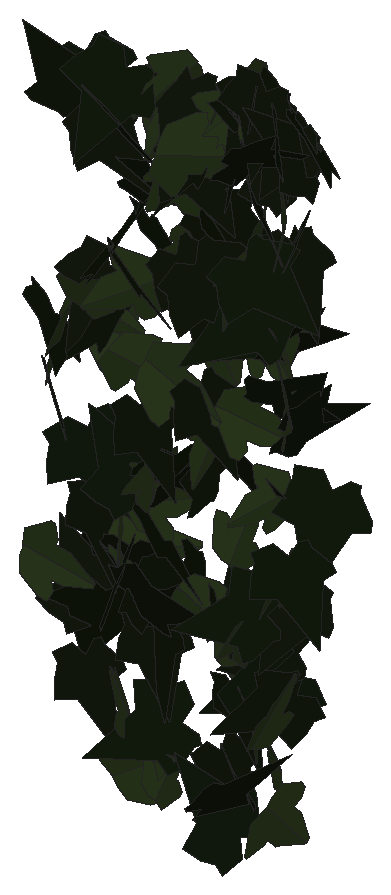
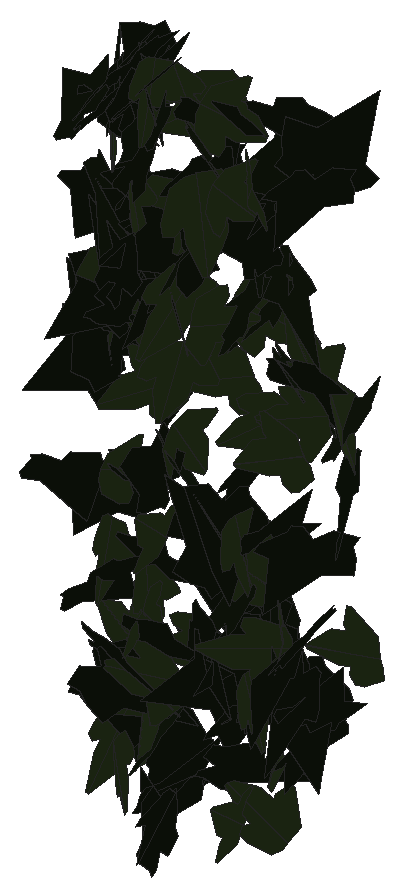
# SketchUp Ruby script. Lengths in inches.
U = 1.inch
M = Sketchup.active_model
def pt(a) = Geom::Point3d.new(a.map { |v| v * U })
def face(e, loops, mat)
  f = e.add_face(loops[0].map { |a| pt(a) })
  loops[1..].each { |l| e.add_face(l.map { |a| pt(a) }).erase! }
  f.material = f.back_material = mat if mat
  f
end
# faces: each face lists its corners as indices into pts; further lists are holes
def faces(e, pts, list, mat = nil) = list.each { |f| face(e, (f[0].is_a?(Array) ? f : [f]).map { |l| l.map { |i| pts[i] } }, mat) }
# xy, xz, yz: faces in a plane at the given z, y or x. An outline is a flat list of corners, or four numbers for a rectangle; further outlines are holes
def ring(l) = l.size == 4 ? [[l[0], l[1]], [l[2], l[1]], [l[2], l[3]], [l[0], l[3]]] : l.each_slice(2).to_a
def flat(e, list, mat, &to3) = list.each { |f| face(e, (f[0].is_a?(Array) ? f : [f]).map { |l| ring(l).map { |u, v| to3.(u, v) } }, mat) }
def xy(e, z, list, mat = nil) = flat(e, list, mat) { |x, y| [x, y, z] }
def xz(e, y, list, mat = nil) = flat(e, list, mat) { |x, z| [x, y, z] }
def yz(e, x, list, mat = nil) = flat(e, list, mat) { |y, z| [x, y, z] }
def lines(e, pts, list) = list.each { |a, b| e.add_line(pt(pts[a]), pt(pts[b])) }
# prism: a flat outline (further loops are holes) pulled along v
def prism(e, loops, v, mat = nil)
  f = face(e, loops, mat); d = Geom::Vector3d.new(v.map { |x| x * U })
  f.pushpull(f.normal.samedirection?(d) ? d.length : -d.length)
end
def box(e, o, s, mat = nil) = prism(e, [[o, [o[0] + s[0], o[1], o[2]], [o[0] + s[0], o[1] + s[1], o[2]], [o[0], o[1] + s[1], o[2]]]], [0, 0, s[2]], mat)
def at(x, y, z, deg = 0) = Geom::Transformation.translation(pt([x, y, z])) * Geom::Transformation.rotation(ORIGIN, Z_AXIS, deg.degrees)
def axes(o, x, y, z) = Geom::Transformation.new([*x, 0, *y, 0, *z, 0, *pt(o).to_a, 1])
def part(name) = M.definitions.add(name)
# library, detail: a bought-in or finely detailed component or shape, given as its bounding box
def library(name, o, s) = part(name).tap { |d| box(d.entities, o, s) }
def detail(e, o, s) = box(e.add_group.entities, o, s)
def put(e, d, t, mat = nil) = e.add_instance(d, t).tap { |i| i.material = mat if mat }
def group(e, t, mat = nil) = e.add_group.tap { |g| g.transformation = t; g.material = mat if mat }.entities
root = M.entities
M.materials.add("efeu1").color = [18, 25, 13]
M.materials.add("efeu2").color = [43, 57, 29]
c1 = part("ivyleaf_10")
p = [[0,0.5,-0.03],[-0.0625,2.02,-0.43],[-0.19,2.01,-0.46],[-0.54,1.05,-0.29],[-0.52,0.625,-0.18],[-0.83,0.76,-0.28],
  [-1.16,0.64,-0.33],[-1.15,0.33,-0.24],[-0.77,-0.39,0.02],[-0.3,-0.51,0.16],[0.04,-0.48,0.23],[-0.02,2.01,-0.4375],
  [-0.06,2.01,-0.43],[0.04,-0.49,0.23],[0.67,-0.49,0.14],[1.38,0.36,-0.2],[1.375,0.51,-0.24],[0.81,0.65,-0.19],
  [0.62,0.59,-0.15],[0.6,1.09,-0.28],[0.5,1.23,-0.31]]
faces(c1.entities,p,[[0,1,2,3,4,5,6,7,8,9,10],[11,12,0,13,14,15,16,17,18,19,20]],"efeu2")
c2 = part("ivyleaf_9")
p = [[1.54,2.16,1.25],[1.36,2.04,1.19],[-0.21,0.99,0.68],[-0.71,1.11,0.82],[-0.85,0.86,0.67],[-0.8,0.17,0.21],
  [-0.9,-0.01,0.1],[-0.67,-0.16,-0.02],[-0.08,-0.08,-0.05],[-0.03,-0.6,-0.4],[0.65,-0.88,-0.66],[0.83,-0.6,-0.49],
  [1.29,-0.42,-0.43],[1.8125,-0.07,-0.26],[1.21,0.44,0.15]]
faces(c2.entities,p,[[0,1,2,3,4,5,6,7,8,9,10,11,12,13,14]],"efeu1")
put(root,c1,axes([549.88,130.77,187.67],[0.2153,-0.80851,0.35731],[-0.00069,0.3676,0.83222],[-0.88394,-0.19722,0.08638]))
put(root,c1,axes([547.04,130.43,204.73],[-0.20339,-0.20216,-0.98043],[0.68566,0.7008,-0.28674],[0.72937,-0.71518,-0.00384]))
put(root,c2,axes([549.13,130.38,205.09],[0.50092,0.40394,0.56191],[0.37323,0.42644,-0.63928],[-0.58276,0.62033,0.07357]))
put(root,c2,axes([549.27,130.88,201.89],[0.22034,-0.57747,-0.68822],[0.24519,0.72037,-0.52594],[0.86429,-0.05715,0.32466]))
put(root,c1,axes([548.82,131.4375,201.4],[0.08871,-0.87143,0.33371],[0.0443,-0.3309,-0.87588],[0.93209,0.09866,0.00987]))
put(root,c2,axes([544.45,131.53,205.83],[-0.79635,-0.51494,-0.12466],[0.10914,0.06079,-0.9483],[0.51845,-0.80376,0.00814]))
put(root,c2,axes([545.1,131.28,190.01],[0.3464,-0.25474,0.81027],[0.68502,-0.43358,-0.42917],[0.50218,0.76717,0.02651]))
put(root,c1,axes([545.3,131.52,199.64],[-0.3442,-0.26523,0.88729],[-0.66707,-0.58559,-0.43382],[0.64237,-0.75023,0.02493]))
put(root,c2,axes([547.65,130.77,201.22],[0.25471,-0.54872,-0.85661],[-0.15872,0.8508,-0.59219],[1.00483,0.27348,0.12359]))
put(root,c1,axes([541.84,131.04,190.28],[0.12516,0.04099,0.9297],[0.89154,0.26368,-0.13165],[-0.26682,0.90027,-0.00377]))
put(root,c2,axes([549.41,131.61,200.25],[-0.90769,-0.27954,0.29998],[-0.2875,-0.08564,-0.94975],[0.29235,-0.95213,-0.00265]))
put(root,c2,axes([548.01,130.67,184.86],[0.23325,0.84885,-0.28298],[0.07285,0.27345,0.88031],[0.89181,-0.24435,0.0021]))
put(root,c2,axes([545,130.55,190.61],[-0.37818,0.2782,-0.85775],[-0.74103,0.4341,0.46752],[0.5138,0.83085,0.04294]))
put(root,c2,axes([549.31,131.46,190.83],[-0.72889,0.02884,0.51759],[-0.51813,-0.01249,-0.72896],[-0.01627,-0.89388,0.02688]))
put(root,c2,axes([548.41,131.43,183.8125],[-0.39425,-0.86849,0.10666],[0.04381,0.09724,0.95379],[-0.87392,0.39667,-0.00031]))
put(root,c1,axes([550.44,130.87,203.55],[0.30747,-0.52133,-0.65044],[-0.24336,0.60694,-0.6015],[0.79727,0.38631,0.06725]))
put(root,c2,axes([544.68,131.05,200.38],[0.77502,-0.30093,-0.2517],[-0.22074,0.12624,-0.83061],[0.32433,0.80503,0.03616]))
put(root,c2,axes([541.79,131.87,197.27],[0.09632,-0.66808,0.62784],[0.21106,-0.59818,-0.6689],[0.89217,0.21364,0.09046]))
put(root,c1,axes([542.41,131.48,197.52],[0.48601,-0.8469,0.10006],[0.04659,-0.08863,-0.97644],[0.85152,0.48823,-0.00368]))
put(root,c2,axes([542.375,130.99,195.75],[0.50052,-0.12141,-0.68792],[-0.66934,0.15881,-0.51503],[0.19989,0.83579,-0.00207]))
put(root,c1,axes([545.95,131.18,197.21],[0.38154,0.15398,0.97579],[0.92976,0.2975,-0.41049],[-0.33382,1.00461,-0.028]))
put(root,c1,axes([550.09,130.9,185.3],[-0.19039,-0.733,-0.64026],[0.21689,0.60404,-0.75602],[0.94878,-0.28517,0.04434]))
put(root,c2,axes([543.29,131.4,187.43],[0.1866,-0.78798,-0.33888],[-0.06518,0.33277,-0.80968],[0.85528,0.19728,0.01223]))
put(root,c2,axes([547.3,131.29,197.09],[0.28273,-0.72917,-0.45243],[-0.1741,0.4177,-0.78201],[0.84028,0.33189,-0.00979]))
put(root,c2,axes([546.625,131.21,200.97],[0.39542,-0.67732,-0.47211],[-0.03229,0.51038,-0.75926],[0.82499,0.34461,0.19657]))
put(root,c1,axes([549.73,131.8125,197.36],[-0.18437,0.10656,0.9668],[0.80848,-0.5303,0.21262],[0.54077,0.82915,0.01174]))
put(root,c2,axes([543.78,131.36,204.5625],[0.88461,-0.46342,0.30091],[0.27313,-0.12703,-0.99855],[0.48032,0.92572,0.01362]))
put(root,c2,axes([542.91,131.59,204.49],[0.49586,0.00518,0.83387],[-0.83093,0.08462,0.49359],[-0.07009,-0.96646,0.04768]))
put(root,c1,axes([544.48,131.53,186.14],[-0.56021,0.64858,0.27437],[0.17947,-0.20754,0.85703],[0.68098,0.58826,-0.00015]))
put(root,c1,axes([543.27,131.49,198.29],[-0.63726,-0.24393,0.44855],[0.46566,0.01659,0.67059],[-0.20943,0.77912,0.12616]))
put(root,c2,axes([544.67,131.16,200.98],[-0.53449,0.90076,-0.00372],[0.00008,-0.00428,-1.0474],[-0.90076,-0.53449,0.00211]))
put(root,c2,axes([550.14,131.55,192.79],[-0.3432,-0.4281,-0.67532],[0.45291,0.50155,-0.54811],[0.65893,-0.5677,0.02501]))
put(root,c1,axes([544.55,131.43,184.31],[-0.49014,-0.18346,0.74154],[0.69282,0.26435,0.52334],[-0.32176,0.84867,-0.00272]))
put(root,c2,axes([548.77,132.23,202.43],[-0.31713,-0.08599,1.04204],[0.23641,-1.06661,-0.01607],[1.0185,0.2208,0.32819]))
put(root,c2,axes([545.875,132.1,186.03],[-0.69274,-0.27828,0.53933],[-0.48329,-0.2421,-0.74568],[0.36708,-0.8439,0.03607]))
put(root,c2,axes([544,131.72,198.49],[-0.86008,0.45628,-0.14401],[0.12256,-0.07625,-0.97357],[-0.46251,-0.86871,0.00981]))
put(root,c1,axes([547.84,131.66,205.57],[0.64046,-0.17967,-0.51993],[-0.51041,0.10351,-0.6645],[0.20516,0.81841,-0.0301]))
put(root,c2,axes([546.96,131.82,204.26],[-0.75488,0.2554,-0.26246],[0.23738,-0.11666,-0.79624],[-0.27887,-0.79065,0.0327]))
put(root,c1,axes([548.64,131.59,190.27],[0.03476,-0.82313,-0.19316],[-0.01652,0.19263,-0.82382],[0.84532,0.03761,-0.00815]))
put(root,c2,axes([543.53,131.6,204.11],[0.32362,-0.67478,-0.53496],[-0.04206,0.55842,-0.72982],[0.86008,0.28121,0.16559]))
put(root,c2,axes([544.89,131.8,195.45],[0.28439,-0.79283,-0.3611],[-0.13006,0.33696,-0.84226],[0.86143,0.31262,-0.00795]))
put(root,c2,axes([549.26,132.36,204.55],[0.01543,-0.12146,0.89187],[0.09367,-0.88694,-0.12241],[0.89522,0.0949,-0.00256]))
put(root,c2,axes([548.2,132.23,205.79],[-0.50467,0.10336,-0.86624],[0.80917,-0.31856,-0.50943],[-0.32605,-0.95057,0.07653]))
put(root,c2,axes([544.53,131.875,192.98],[-0.48463,-0.68658,0.17349],[0.0965,0.14423,0.84038],[-0.70156,0.49412,-0.00424]))
put(root,c1,axes([547.04,132.26,195.52],[-0.08739,-0.70219,0.49403],[0.16901,-0.50094,-0.68211],[0.84177,0.02768,0.18824]))
put(root,c2,axes([548.6,132.42,206.16],[-0.08248,-0.86156,0.18638],[0.00251,-0.18743,-0.86527],[0.88149,-0.08008,0.0199]))
put(root,c2,axes([548.85,132.1,198.96],[0.44175,-0.55624,0.5064],[-0.31219,0.39873,0.71031],[-0.68438,-0.54093,0.00285]))
put(root,c2,axes([547.6875,131.42,199.9],[0.05818,-0.19803,-0.85883],[-0.2863,0.80977,-0.20612],[0.83357,0.29195,-0.01086]))
put(root,c2,axes([549.31,131.99,197.12],[0.88785,0.35219,-0.14803],[0.12722,0.08058,0.95475],[0.36023,-0.89649,0.02766]))
put(root,c1,axes([548.97,132.56,193.92],[-0.15855,-0.1143,0.80153],[-0.07362,-0.81134,-0.13026],[0.80629,-0.09655,0.14573]))
put(root,c2,axes([543.57,131.875,189.3125],[0.44343,0.65671,-0.6723],[-0.37509,-0.55794,-0.7924],[-0.86172,0.5808,-0.00104]))
put(root,c1,axes([543.57,132.52,190.8],[-0.13446,0.2921,-0.82646],[0.3256,-0.75965,-0.32146],[-0.81384,-0.35218,0.00793]))
put(root,c1,axes([545.66,132.58,205.78],[-0.09236,-0.50742,0.7116],[-0.17013,-0.69144,-0.51512],[0.85727,-0.19189,-0.02556]))
put(root,c1,axes([549.45,131.98,199.77],[-0.61986,-0.61374,-0.08379],[0.05805,0.06046,-0.87229],[0.61671,-0.62257,-0.00211]))
put(root,c1,axes([548.07,131.67,196.46],[0.28351,0.20634,0.86985],[0.61896,0.61314,-0.34718],[-0.64506,0.67902,0.04917]))
put(root,c2,axes([549.46,132.59,187.91],[-0.10826,-0.07072,-0.82973],[-0.15743,-0.81989,0.09042],[-0.81773,0.16721,0.09244]))
put(root,c1,axes([544.2,131.84,196.875],[-0.4389,-0.16426,-0.72473],[0.68405,0.23956,-0.46855],[0.29035,-0.8127,0.00837]))
put(root,c2,axes([546.02,132.42,205.63],[-0.69596,-0.43216,-0.32261],[0.27749,0.16466,-0.81919],[0.46243,-0.74921,0.00605]))
put(root,c2,axes([544.27,132.02,202.24],[0.57296,-0.13827,0.57344],[0.55953,-0.1257,-0.58937],[0.18675,0.80082,0.0065]))
put(root,c2,axes([543.15,132.45,198.91],[-0.76947,-0.31414,-0.21104],[0.19197,0.08809,-0.83108],[0.32614,-0.793,-0.00872]))
put(root,c2,axes([545.06,132.39,188.55],[-0.4678,-0.08667,-0.72352],[0.72076,0.07151,-0.47458],[0.10725,-0.85861,0.03351]))
put(root,c1,axes([546.25,131.87,203.03],[-0.59504,-0.60988,-0.48951],[0.32396,0.3676,-0.8518],[0.71177,-0.67717,-0.02153]))
put(root,c2,axes([549.66,132.3,201.9],[-0.4015,-0.35129,-0.73442],[0.6341,0.37863,-0.52776],[0.51058,-0.74647,0.07792]))
put(root,c2,axes([548.1,132.87,205.45],[-0.23026,-0.66515,0.52656],[-0.0111,-0.5432,-0.69103],[0.84827,-0.18767,0.13389]))
put(root,c2,axes([549.89,132.6,204.48],[0.07188,-0.90825,-0.00172],[0.00906,-0.00101,0.91105],[-0.90821,-0.07189,0.00895]))
put(root,c2,axes([547.44,131.82,194.39],[-0.54665,0.67911,0.44936],[-0.2715,0.35826,-0.87171],[-0.76772,-0.61025,-0.01169]))
put(root,c1,axes([548.52,132.34,198.79],[0.4058,-0.04833,0.8407],[0.83765,-0.0726,-0.4085],[0.08641,0.93069,0.0118]))
put(root,c1,axes([545.6,131.64,184.23],[0.0663,0.49334,-0.68548],[0.0995,0.67824,0.49775],[0.83867,-0.11946,-0.00487]))
put(root,c2,axes([548.43,132.82,204.98],[-0.15026,0.0726,0.87994],[-0.50317,-0.7405,-0.02483],[0.72552,-0.49853,0.16503]))
put(root,c2,axes([544.78,132.26,191.89],[0.79009,-0.59008,-0.12677],[-0.09836,0.08016,-0.98611],[0.59547,0.79618,0.00532]))
put(root,c2,axes([549.72,132.22,204.17],[-0.81542,-0.22777,-0.38594],[-0.37359,-0.09706,0.84661],[-0.24751,0.89691,-0.00639]))
put(root,c2,axes([544.97,131.74,190.23],[0.13576,-0.00107,-0.81488],[-0.33059,0.75501,-0.05606],[0.74481,0.33531,0.12365]))
put(root,c1,axes([544.93,132.44,193.44],[-0.04396,-0.89604,0.03976],[-0.00277,-0.03967,-0.89712],[0.89692,-0.04404,-0.00082]))
put(root,c2,axes([544.71,132.5625,188.375],[0.0614,-0.83782,-0.22154],[-0.04297,0.21888,-0.83966],[0.86555,0.0703,-0.02597]))
put(root,c2,axes([546.2,132.24,203.83],[0.20092,-0.75038,-0.60078],[-0.15154,0.58136,-0.7768],[0.94923,0.25165,0.00315]))
put(root,c1,axes([548.45,132.37,202.12],[0.32828,-0.83126,-0.13869],[-0.0206,0.14088,-0.89316],[0.8425,0.32734,0.0322]))
put(root,c2,axes([542.71,132.26,193.84],[-0.13402,-0.63271,-0.7364],[0.18437,0.71327,-0.64639],[0.95321,-0.22692,0.02148]))
put(root,c2,axes([542.76,132.37,188.55],[-0.61914,-0.5843,0.22468],[0.16544,0.15205,0.85131],[-0.60375,0.64086,0.00287]))
put(root,c2,axes([550.13,131.62,196.73],[0.34409,0.49996,0.73401],[0.43616,0.59058,-0.60673],[-0.77363,0.55532,-0.01559]))
put(root,c1,axes([544.41,132.29,192.2],[-0.3229,-0.16237,0.88721],[0.81547,0.3501,0.36087],[-0.38539,0.87684,0.02021]))
put(root,c2,axes([549.74,131.69,201.44],[-0.08106,0.62413,0.77413],[-0.07177,0.771,-0.62913],[-0.9918,-0.1068,-0.01775]))
put(root,c2,axes([548.83,133.02,199.13],[-0.61682,-0.41882,0.51172],[-0.43713,-0.26683,-0.74529],[0.49618,-0.75573,-0.02045]))
put(root,c2,axes([549.09,133.15,204.92],[-0.23887,-0.7398,0.46488],[-0.01798,-0.47768,-0.76941],[0.87356,-0.21213,0.11129]))
put(root,c2,axes([546.89,132.83,199.96],[-0.3895,0.0016,-0.76927],[0.74903,-0.1957,-0.37966],[-0.1753,-0.83975,0.08701]))
put(root,c1,axes([546.07,132.45,189.86],[-0.4727,-0.01443,-0.69725],[0.69418,-0.09048,-0.46875],[-0.06685,-0.8375,0.06266]))
put(root,c1,axes([542.54,132.49,197.74],[-0.3058,0.00048,-0.79574],[0.79243,-0.07754,-0.30458],[-0.07255,-0.84894,0.02737]))
put(root,c2,axes([547.68,133.03,204.48],[0.67163,-0.56394,-0.15563],[0.15167,-0.061,0.87557],[-0.56502,-0.68672,0.05003]))
put(root,c2,axes([546.6,132.95,201.14],[0.38755,-0.69043,0.3946],[0.17362,-0.35491,-0.79151],[0.77605,0.42419,-0.01998]))
put(root,c2,axes([542.48,132.85,191.39],[0.24106,-0.84777,-0.03134],[-0.00575,0.03095,-0.88138],[0.84833,0.24111,0.00293]))
put(root,c2,axes([547.2,132.78,194.36],[0.40828,-0.32089,0.63116],[0.47584,-0.41516,-0.51889],[0.52432,0.62665,-0.02057]))
put(root,c1,axes([547.86,131.97,192.15],[0.16692,0.55295,-0.67549],[0.09586,0.67195,0.57375],[0.86767,-0.18061,0.06656]))
put(root,c1,axes([549.39,132.23,191.73],[0.01056,-0.71991,-0.55145],[-0.02302,0.55109,-0.71989],[0.90655,0.02238,-0.01185]))
put(root,c1,axes([547.7,132.98,190.29],[0.00593,0.62166,-0.62218],[0.02795,-0.62201,-0.62123],[-0.87908,-0.01558,-0.02394]))
put(root,c2,axes([545.62,132.37,194.03],[0.28996,0.76052,-0.38598],[-0.14251,-0.35874,-0.81391],[-0.84087,0.32305,0.00484]))
put(root,c1,axes([547.83,132.92,186.12],[-0.56836,0.36184,0.57297],[0.43953,-0.37236,0.67114],[0.51579,0.71602,0.05947]))
put(root,c2,axes([548.99,132.99,188.19],[-0.01197,-0.04915,-0.96158],[-0.54657,-0.79135,0.04726],[-0.79266,0.5464,-0.01806]))
put(root,c2,axes([549.26,133.27,190.8125],[-0.38793,-0.8102,0.2561],[-0.0944,-0.23869,-0.89811],[0.84445,-0.39888,0.01725]))
put(root,c2,axes([544.27,132.98,200.46],[0.49046,-0.67686,0.32212],[0.18446,-0.26412,-0.83586],[0.72655,0.52397,-0.00523]))
put(root,c1,axes([546.06,132.74,203.23],[-0.46192,-0.9782,0.03968],[-0.01652,-0.03608,-1.08178],[0.97887,-0.46221,0.00047]))
put(root,c2,axes([549.41,132,199.03],[0.41876,0.55323,0.53455],[0.31135,0.43467,-0.69376],[-0.70347,0.5217,0.01116]))
put(root,c1,axes([546.9,132.5625,197.98],[-0.5227,-0.63536,-0.25479],[0.1718,0.18856,-0.82264],[0.66263,-0.55007,0.0123]))
put(root,c2,axes([547.09,133.1,186.89],[0.34986,-0.77664,0.20114],[0.11295,-0.16957,-0.85119],[0.79427,0.3662,0.03244]))
put(root,c2,axes([544.02,132.46,190.58],[0.69622,0.5089,-0.45215],[-0.37953,-0.24674,-0.86211],[-0.56514,0.79265,0.02193]))
put(root,c1,axes([547.71,132.55,206.11],[-0.11998,-0.80416,-0.39552],[0.04638,0.39294,-0.81299],[0.89496,-0.12816,-0.01089]))
put(root,c2,axes([549.46,133.3,204.79],[0.16813,-0.57886,0.64341],[0.34844,-0.5547,-0.5901],[0.79224,0.36682,0.12299]))
put(root,c2,axes([546.93,133.32,183.78],[0.02812,-0.23036,0.88742],[0.38077,-0.80471,-0.22096],[0.83402,0.37516,0.07096]))
put(root,c2,axes([542.22,132.78,204.99],[-0.04014,-0.66698,-0.60192],[0.05108,0.59985,-0.66809],[0.89697,-0.06401,0.01111]))
put(root,c1,axes([544.74,133.39,204.04],[-0.0863,-0.58021,0.63508],[0.16489,-0.63759,-0.5601],[0.84427,0.06522,0.17431]))
put(root,c2,axes([547.73,133.04,189.61],[-0.69284,0.12511,0.53559],[-0.53581,0.04091,-0.70268],[-0.12415,-0.87476,0.04374]))
put(root,c2,axes([546.8125,132.8125,185.11],[0.24925,-0.69712,-0.46598],[-0.16203,0.43693,-0.74033],[0.82272,0.29725,-0.00463]))
put(root,c2,axes([545.3125,132.64,192.67],[0.31941,0.87127,0.13479],[-0.06946,-0.11805,0.92765],[0.8789,-0.32596,0.02432]))
put(root,c1,axes([545.35,133.47,199.98],[0.06031,0.2385,-0.84343],[-0.42829,-0.72961,-0.23694],[-0.76474,0.42742,0.06618]))
put(root,c2,axes([546.27,132.69,190.29],[0.09922,0.04757,-0.94181],[-0.93547,-0.11458,-0.10434],[-0.11904,0.94007,0.03494]))
put(root,c2,axes([550.15,133.28,194.05],[-0.6364,-0.66708,-0.29739],[0.206,0.21449,-0.92196],[0.70072,-0.66891,0.00094]))
put(root,c1,axes([547.0625,132.95,188.53],[-0.13707,-0.00409,-0.96092],[0.94528,-0.17506,-0.1341],[-0.17274,-0.95473,0.0287]))
put(root,c2,axes([542.74,132.66,190.01],[0.83169,-0.00458,-0.48617],[-0.48618,-0.00139,-0.83169],[0.00325,0.96336,-0.00351]))
put(root,c1,axes([548.86,132.55,185.47],[0.36656,-0.22428,-0.77737],[-0.39717,0.69364,-0.38741],[0.70488,0.50747,0.18597]))
put(root,c2,axes([546.51,132.78,201.74],[0.07595,-0.0471,-0.905],[0.59437,0.68814,0.01406],[0.68408,-0.59267,0.08826]))
put(root,c1,axes([543.73,133.375,204.44],[0.46422,-0.2594,0.66136],[0.58519,-0.30832,-0.53168],[0.4028,0.74688,0.01022]))
put(root,c1,axes([546.59,132.63,200.21],[-0.36094,-0.74129,-0.69095],[0.39038,0.57515,-0.82098],[0.93516,-0.5262,0.07604]))
put(root,c2,axes([545.17,132.47,189.12],[0.47992,0.31849,0.65235],[0.53758,0.36962,-0.57594],[-0.48785,0.7206,0.00709]))
put(root,c2,axes([548.15,133.4,200.18],[-0.0795,-0.00027,0.88074],[0.48278,-0.73964,0.04335],[0.73663,0.48472,0.06664]))
put(root,c1,axes([542.8125,132.97,196.6875],[0.36032,0.11434,0.88818],[0.85143,0.25294,-0.37797],[-0.2775,0.92451,-0.00643]))
put(root,c1,axes([543.99,133.21,189.4],[0.1483,-0.84263,0.03176],[0.0054,-0.03129,-0.85558],[0.84321,0.14839,-0.0001]))
put(root,c1,axes([543.67,132.7,190.53],[0.01173,-0.09017,-0.96091],[0.88645,0.38104,-0.02493],[0.38167,-0.88221,0.08744]))
put(root,c2,axes([549.08,133.08,188.88],[-0.79756,0.37027,0.39319],[-0.36009,0.15809,-0.87928],[-0.40253,-0.87505,0.00752]))
